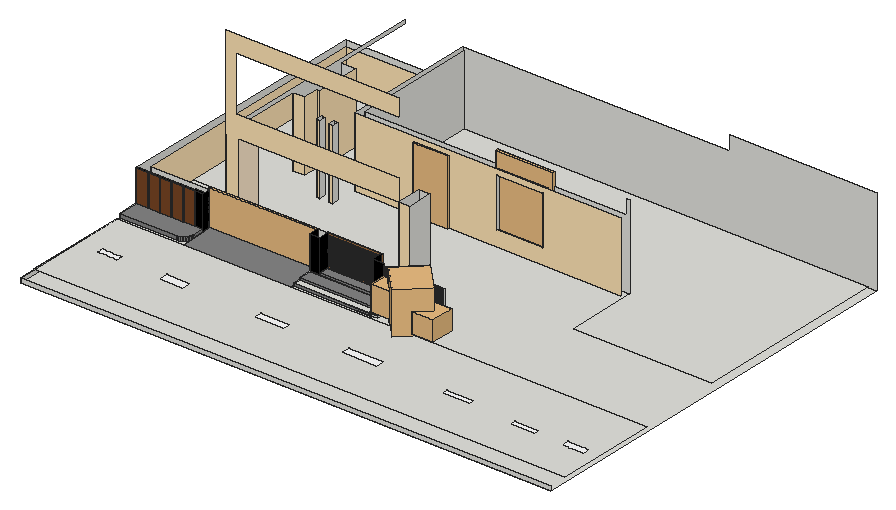
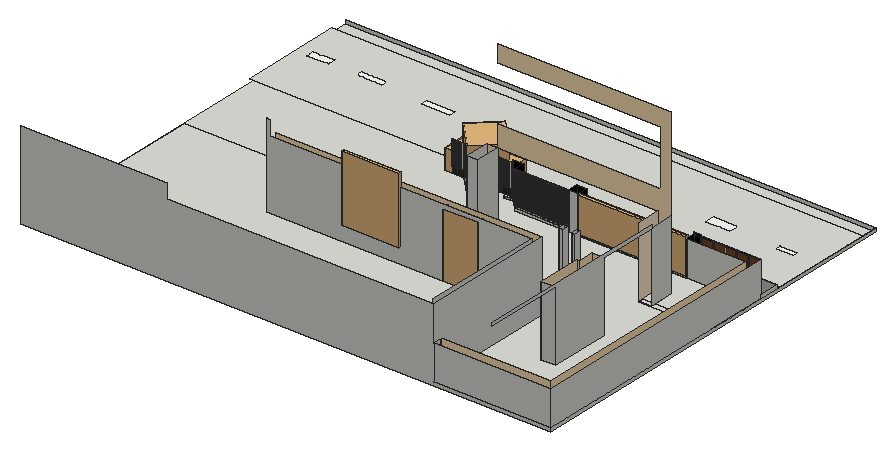
# SketchUp Ruby script. Lengths in inches.
U = 1.inch
M = Sketchup.active_model
def pt(a) = Geom::Point3d.new(a.map { |v| v * U })
def face(e, loops, mat)
  f = e.add_face(loops[0].map { |a| pt(a) })
  loops[1..].each { |l| e.add_face(l.map { |a| pt(a) }).erase! }
  f.material = f.back_material = mat if mat
  f
end
# faces: each face lists its corners as indices into pts; further lists are holes
def faces(e, pts, list, mat = nil) = list.each { |f| face(e, (f[0].is_a?(Array) ? f : [f]).map { |l| l.map { |i| pts[i] } }, mat) }
# xy, xz, yz: faces in a plane at the given z, y or x. An outline is a flat list of corners, or four numbers for a rectangle; further outlines are holes
def ring(l) = l.size == 4 ? [[l[0], l[1]], [l[2], l[1]], [l[2], l[3]], [l[0], l[3]]] : l.each_slice(2).to_a
def flat(e, list, mat, &to3) = list.each { |f| face(e, (f[0].is_a?(Array) ? f : [f]).map { |l| ring(l).map { |u, v| to3.(u, v) } }, mat) }
def xy(e, z, list, mat = nil) = flat(e, list, mat) { |x, y| [x, y, z] }
def xz(e, y, list, mat = nil) = flat(e, list, mat) { |x, z| [x, y, z] }
def yz(e, x, list, mat = nil) = flat(e, list, mat) { |y, z| [x, y, z] }
def lines(e, pts, list) = list.each { |a, b| e.add_line(pt(pts[a]), pt(pts[b])) }
# prism: a flat outline (further loops are holes) pulled along v
def prism(e, loops, v, mat = nil)
  f = face(e, loops, mat); d = Geom::Vector3d.new(v.map { |x| x * U })
  f.pushpull(f.normal.samedirection?(d) ? d.length : -d.length)
end
def box(e, o, s, mat = nil) = prism(e, [[o, [o[0] + s[0], o[1], o[2]], [o[0] + s[0], o[1] + s[1], o[2]], [o[0], o[1] + s[1], o[2]]]], [0, 0, s[2]], mat)
def at(x, y, z, deg = 0) = Geom::Transformation.translation(pt([x, y, z])) * Geom::Transformation.rotation(ORIGIN, Z_AXIS, deg.degrees)
def axes(o, x, y, z) = Geom::Transformation.new([*x, 0, *y, 0, *z, 0, *pt(o).to_a, 1])
def part(name) = M.definitions.add(name)
# library, detail: a bought-in or finely detailed component or shape, given as its bounding box
def library(name, o, s) = part(name).tap { |d| box(d.entities, o, s) }
def detail(e, o, s) = box(e.add_group.entities, o, s)
def put(e, d, t, mat = nil) = e.add_instance(d, t).tap { |i| i.material = mat if mat }
def group(e, t, mat = nil) = e.add_group.tap { |g| g.transformation = t; g.material = mat if mat }.entities
root = M.entities
M.materials.add("Color_000").color = [255, 255, 255]
M.materials.add("Material__1").color = [95, 70, 46]
M.materials.add("Material__2").color = [150, 168, 104]
M.materials.add("[0029_BlanchedAlmond]").color = [255, 235, 205]
M.materials.add("[0032_Moccasin]").color = [255, 228, 181]
M.materials.add("[0136_Charcoal]").color = [35, 35, 35]
M.materials.add("[0137_Black]").color = [0, 0, 0]
M.materials.add("[Tile Grey]").color = [132, 132, 132]
M.materials.add("[Wood Floor Light]").color = [204, 176, 127]
M.materials.add("[Wood Floor]").color = [155, 105, 61]
M.materials.add("[Wood Veneer 01]").color = [120, 70, 37]
M.materials.add("wire_2").color = [244, 244, 244]
M.materials.add("wire_5").color = [232, 232, 232]
c1 = library("Group\#82",[0,0,0],[156.52,4.3,60.67])
c2 = library("door (1)",[38.93,25.48,0],[40,9.94,82.68])
c3 = part("Group\#65")
box(c3.entities,[0,0,0],[1.57,1.97,82.68])
c4 = library("Potted plant on stand",[0,0,0],[37.88,32.09,49.42])
c5 = part("Untitled (5)")
xy(c5.entities,0,[[[158.81,26.5625,306.06,993.3125],[226.57,518.17,239.57,583.92],[225.28,357.51,237.28,411.51],[222.61,182.28,236.36,226.53],[239.71,931.55,251.46,972.3],[233.64,703.93,242.14,755.18],[240.05,835.03,248.8,880.53],[222.04,66.5,231.29,100.5]]])
xy(c5.entities,0,[[222.04,66.5,231.29,100.5],[222.61,182.28,236.36,226.53],[225.28,357.51,237.28,411.51],[226.57,518.17,239.57,583.92],[233.64,703.93,242.14,755.18],
  [240.05,835.03,248.8,880.53],[239.71,931.55,251.46,972.3]],"Color_000")
c6 = library("Cylinder004__30___50_",[-997.48,-49.45,708.79],[29.81,29.81,30.61])
c7 = library("Group\#401",[-996.8,-48.73,736.67],[28.51,28.38,4.73])
c8 = library("Group\#404",[-994.36,-46.95,735.88],[24.38,25.9,6.88])
c9 = library("Group\#388",[-1022.2,-71.69,736.68],[86.94,78.77,45.64])
c10 = library("3 door",[0,0,0],[74.8,3.9375,43.31])
c11 = library("panneau+shadow+blanc+bourdon+naturel",[-47.99,-1.29,1.53],[97.82,5.86,114.18])
c12 = library("Palm",[82.2,-9.29,-2.36],[51.18,55.77,65.42])
c13 = library("Pinch Pot",[-27.95,-27.95,0],[55.9,55.9,47.42])
c14 = library("Group\#386",[-915.9375,-34.5,735.6],[41.04,40.85,6.81])
c15 = library("Group\#403",[-912.1,-32.49,735.82],[33.14,36.63,9.55])
c16 = part("Potted palm")
put(c16.entities,c12,axes([3796.42,-10488.37,43.97],[0,116.51338,0],[-116.51338,0,0],[0,0,116.51338]))
put(c16.entities,c13,axes([1647.67,1801.1875,0],[0,30.58476,0],[-30.58476,0,0],[0,0,45.1095]))
put(c16.entities,c14,axes([32580.48,2279.8125,-23417.78],[34.48768,0,0],[0,34.48768,0],[0,0,34.48768]),"Material__1")
put(c16.entities,c15,axes([32580.48,2279.8125,-23417.78],[34.48768,0,0],[0,34.48768,0],[0,0,34.48768]),"wire_5")
c17 = library("Agrupar\#177",[0,0,0],[36.52,33.08,30.88])
c18 = library("Agrupar\#154",[0,0,0],[41.26,44.6,38.97])
xy(root,0,[[0,84.05,912.4375,784.05]])
xy(root,5.8125,[[0,431.86,124.125,440.22]])
xy(root,6.6875,[[298.71,289.39,114.03,290.125,114.12,311.98,114.13,312.05,114.13,314.23,114.2,333.31,114.27,349.54,298.96,349.54],[298.96,298.09,315.7,332.68],[315.7,298.09,408.98,332.68],[408.98,298.09,430.8,298.09,429.97,299.48,429.25,300.94,428.64,302.43,428.13,303.97,427.73,305.54,427.45,307.14,427.28,308.75,427.22,310.37,427.22,331.81,408.98,331.81],[430.8,298.09,429.97,299.48,429.25,300.94,428.64,302.43,428.13,303.97,427.73,305.54,427.45,307.14,427.28,308.75,427.22,310.37,427.22,331.81,443.3,331.81,443.3,298.09],
  [114.12,311.98,114.13,314.23,114.13,312.05],[298.96,332.68,315.7,349.54],[114.2,333.31,114.27,349.54,114.2,349.54],[114.27,349.54,298.96,349.54,114.27,350.28],[101.6875,397.92,124.125,431.86],
  [101.6875,431.86,124.125,440.22],[666.61,440.22,904.08,440.22,904.08,775.6875,209.98,775.6875,209.98,562.07,666.61,562.07],[101.6875,542.92,121.5,551.1875],[101.6875,551.1875,121.5,569.92]])
xy(root,9.8125,[[298.96,298.09,443.3,298.09,443.3,331.81,430.42,331.81,430.42,310.31,298.96,310.31],[298.96,310.31,315.7,332.68],[315.7,310.31,408.98,332.68],[408.98,310.31,430.42,331.81],[315.7,332.68,408.98,349.54]])
xy(root,12.75,[[0,297.16,98.1875,297.16,100.36,297.31,102.5,297.75,104.55,298.48,106.49,299.49,108.27,300.74,109.87,302.23,111.24,303.93,112.375,305.79,113.25,307.79,113.83,309.89,114.12,311.98,114.13,314.23,114.2,333.31,101.04,333.31,101.04,334.06,100.22,334.06,100.22,333.31,80.99,333.31,80.99,334.06,80.18,334.06,80.18,333.31,60.95,333.31,60.95,334.06,60.13,334.06,60.13,333.31,40.9,333.31,40.9,334.06,40.09,334.06,40.09,333.31,20.86,333.31,20.86,334.06,20.04,334.06,20.04,333.31,0,333.31]],"[Tile Grey]")
xy(root,13.1875,[[315.7,332.68,408.98,349.54]])
xy(root,13.1875,[[298.96,310.31,430.42,310.31,430.42,331.81,408.98,331.81,408.98,332.68,298.96,332.68]],"[Tile Grey]")
xy(root,16.5625,[[315.7,332.68,408.98,349.54]],"[Tile Grey]")
xy(root,32.4,[[446,551.1875,524.68,562.07]])
xz(root,84.05,[[0,0,912.4375,6.6875]])
xz(root,297.16,[[0,6.6875,98.1875,12.75]],"[Tile Grey]")
xz(root,298.09,[[430.8,6.6875,443.3,9.8125]])
xz(root,298.09,[[298.96,6.6875,430.8,9.8125]],"[Tile Grey]")
xz(root,301.86,[[440.93,11.9375,442.89,26],[442.89,11.9375,443.8,26],[443.8,11.9375,445.77,26],[445.77,11.9375,446.68,26],[446.68,11.9375,448.64,26],
  [448.64,11.9375,449.55,26],[449.55,11.9375,451.52,26],[451.52,11.9375,452.37,26],[452.37,11.9375,454.33,26],[454.33,11.9375,455.18,26],
  [455.18,11.9375,457.14,26],[457.14,11.9375,457.99,26],[457.99,11.9375,459.95,26],[459.95,11.9375,460.8,26],[460.8,11.9375,462.77,26],
  [462.77,11.9375,463.62,26],[463.62,11.9375,465.58,26],[465.58,11.9375,466.43,26],[466.43,11.9375,468.39,26],[468.39,11.9375,469.24,26],
  [469.24,11.9375,471.2,26],[471.2,11.9375,472.05,26],[472.05,11.9375,474.02,26],[474.02,11.9375,474.87,26],[474.87,11.9375,476.83,26],
  [476.83,11.9375,477.68,26],[477.68,11.9375,479.64,26],[479.64,11.9375,480.49,26],[480.49,11.9375,482.45,26],[482.45,11.9375,483.3,26],
  [483.3,11.9375,485.27,26],[485.27,11.9375,486.12,26],[486.12,11.9375,488.08,26],[488.08,11.9375,488.93,26],[488.93,11.9375,490.89,26],
  [490.89,11.9375,491.74,26],[491.74,11.9375,493.7,26],[493.7,11.9375,494.55,26],[494.55,11.9375,496.52,26],[496.52,11.9375,497.37,26],
  [497.37,11.9375,499.33,26],[499.33,11.9375,500.18,26],[500.18,11.9375,502.14,26],[502.14,11.9375,502.99,26],[502.99,11.9375,504.95,26],
  [504.95,11.9375,505.8,26],[505.8,11.9375,507.77,26],[507.77,11.9375,508.62,26],[508.62,11.9375,510.58,26],[510.58,11.9375,511.43,26],
  [511.43,11.9375,513.39,26],[513.39,11.9375,514.24,26],[514.24,11.9375,516.2,26],[516.2,11.9375,517.05,26],[517.05,11.9375,519.02,26],
  [519.02,11.9375,520.39,26],[520.39,11.9375,522.35,26],[522.35,11.9375,523.72,26],[523.72,11.9375,525.68,26],[525.68,11.9375,527.06,26],
  [527.06,11.9375,529.02,26],[529.02,11.9375,530.39,26],[530.39,11.9375,532.35,26]],"[Wood Veneer 01]")
xz(root,310.31,[[298.96,9.8125,430.42,13.1875]],"[Tile Grey]")
xz(root,328.88,[[464.85,11.9375,475.34,26]],"[0136_Charcoal]")
xz(root,328.94,[[462.96,11.9375,464.85,26]])
xz(root,328.94,[[452.48,11.9375,462.96,26],[475.34,11.9375,479.46,26]],"[0136_Charcoal]")
xz(root,329,[[430.83,11.9375,434.09,26],[434.09,11.9375,438.21,26],[438.21,11.9375,442.34,26],[442.34,11.9375,446.46,26],[446.46,11.9375,450.59,26],
  [450.59,11.9375,452.48,26],[479.46,11.9375,483.59,26],[483.59,11.9375,487.71,26],[487.71,11.9375,491.84,26],[491.84,11.9375,495.96,26],
  [495.96,11.9375,500.09,26],[500.09,11.9375,504.21,26],[504.21,11.9375,508.34,26],[508.34,11.9375,512.46,26],[512.46,11.9375,516.59,26],
  [516.59,11.9375,520.71,26],[520.71,11.9375,524.84,26],[524.84,11.9375,528.96,26],[528.96,11.9375,533.09,26]],"[0136_Charcoal]")
xz(root,331.81,[[408.98,6.6875,427.22,9.8125],[427.22,6.6875,443.3,9.8125],[408.98,9.8125,427.22,13.1875],[427.22,9.8125,430.42,13.1875]])
xz(root,331.81,[[408.98,13.1875,427.22,70.8125]],"[0137_Black]")
xz(root,332.49,[[468.47,26,471.72,66.6875]],"[Wood Veneer 01]")
xz(root,332.56,[[456.09,26,459.35,66.6875],[464.34,26,467.6,66.6875],[472.59,26,475.85,66.6875]],"[Wood Veneer 01]")
xz(root,332.62,[[427.22,26,430.47,66.6875],[431.34,26,434.6,66.6875],[435.47,26,438.72,66.6875],[439.59,26,442.85,66.6875],[443.72,26,446.97,66.6875],
  [447.84,26,451.1,66.6875],[451.97,26,455.22,66.6875],[460.22,26,463.47,66.6875],[476.72,26,479.97,66.6875],[480.84,26,484.1,66.6875],
  [484.97,26,488.22,66.6875],[489.09,26,492.35,66.6875],[493.22,26,496.47,66.6875],[497.34,26,500.6,66.6875],[501.47,26,504.72,66.6875],
  [505.59,26,508.85,66.6875],[509.72,26,512.97,66.6875],[513.84,26,517.1,66.6875],[517.97,26,521.22,66.6875],[522.09,26,525.35,66.6875],
  [526.22,26,529.47,66.6875]],"[Wood Veneer 01]")
xz(root,332.68,[[298.96,6.6875,315.7,9.8125],[315.7,6.6875,408.98,9.8125],[298.96,9.8125,315.7,13.1875],[315.7,9.8125,408.98,13.1875]])
xz(root,332.68,[[298.96,13.1875,315.7,70.8125]],"[0137_Black]")
xz(root,332.68,[[315.7,13.1875,408.98,16.5625]],"[Tile Grey]")
xz(root,333.31,[[101.04,12.75,114.2,66.6875]],"[0137_Black]")
xz(root,333.31,[[0,12.75,20.04,66.6875],[20.86,12.75,40.09,66.6875],[40.9,12.75,60.13,66.6875],[60.95,12.75,80.18,66.6875],[80.99,12.75,100.22,66.6875],
  [430.47,26,431.34,66.6875],[434.6,26,435.47,66.6875],[438.72,26,439.59,66.6875],[442.85,26,443.72,66.6875],[446.97,26,447.84,66.6875],
  [451.1,26,451.97,66.6875],[455.22,26,456.09,66.6875],[459.35,26,460.22,66.6875],[463.47,26,464.34,66.6875],[467.6,26,468.47,66.6875],
  [471.72,26,472.59,66.6875],[475.85,26,476.72,66.6875],[479.97,26,480.84,66.6875],[484.1,26,484.97,66.6875],[488.22,26,489.09,66.6875],
  [492.35,26,493.22,66.6875],[496.47,26,497.34,66.6875],[500.6,26,501.47,66.6875],[504.72,26,505.59,66.6875],[508.85,26,509.72,66.6875],
  [512.97,26,513.84,66.6875],[517.1,26,517.97,66.6875],[521.22,26,522.09,66.6875],[525.35,26,526.22,66.6875],[529.47,26,530.34,66.6875]],"[Wood Veneer 01]")
xz(root,334.06,[[20.04,12.75,20.86,12.75,20.86,66.6875,40.09,66.6875,40.09,12.75,40.9,12.75,40.9,66.6875,60.13,66.6875,60.13,12.75,60.95,12.75,60.95,66.6875,80.18,66.6875,80.18,12.75,80.99,12.75,80.99,66.6875,100.22,66.6875,100.22,12.75,101.04,12.75,101.04,66.6875,114.2,66.6875,114.2,70.8125,101.1875,70.8125,101.1875,68.25,0,68.25,0,66.6875,20.04,66.6875]],"[0137_Black]")
xz(root,349.54,[[12.79,6.6875,114.2,66.6875],[298.96,6.6875,315.7,70.8125],[315.7,6.6875,408.98,9.8125],[315.7,9.8125,408.98,13.1875],[315.7,13.1875,408.98,16.5625]])
xz(root,397.92,[[101.6875,6.6875,124.125,6.6875,124.125,126.6875,400.76,126.6875,400.76,163.5625,118.89,163.5625,118.89,258.66,400.76,258.66,400.76,287.5625,101.6875,287.5625],[400.76,6.6875,418.84,126.6875]],"[0032_Moccasin]")
xz(root,440.22,[[400.76,6.6875,418.84,126.6875]])
xz(root,506.17,[[171.55,6.6875,177.8,126.6875],[192.11,6.6875,199.48,126.6875]],"[0032_Moccasin]")
xz(root,517.35,[[171.55,6.6875,177.8,126.6875],[192.11,6.6875,199.48,126.6875]])
xz(root,542.92,[[101.6875,6.6875,121.5,126.6875]],"[0032_Moccasin]")
xz(root,551.1875,[[[201.625,6.6875,303.76,6.6875,303.76,118.5,363.88,118.5,363.88,6.6875,660.05,6.6875,660.05,126.6875,201.625,126.6875],[446,32.4,524.68,117.59]]],"[0032_Moccasin]")
xz(root,562.07,[[[209.98,6.6875,209.98,126.6875,660.05,126.6875,660.05,151.4375,666.61,151.4375,666.61,6.6875,363.88,6.6875,363.88,118.5,303.76,118.5,303.76,6.6875],[446,32.4,524.68,117.59]]])
xz(root,569.92,[[121.5,6.6875,126.375,126.6875]],"[0032_Moccasin]")
xz(root,646.79,[[101.6875,6.6875,126.375,126.6875]])
xz(root,768.3,[[12.79,6.6875,201.625,66.6875]],"[0032_Moccasin]")
xz(root,784.05,[[0,0,0,6.6875,201.625,6.6875,201.625,126.6875,660.05,126.6875,660.05,151.4375,912.4375,151.4375,912.4375,0],[0,6.6875,201.625,66.6875]])
yz(root,0,[[84.05,0,84.05,5.8125,440.22,5.8125,440.22,6.6875,784.05,6.6875,784.05,0],[84.05,5.8125,84.05,6.6875,144.1,6.6875,170.97,5.8125],[170.97,5.8125,144.1,6.6875,297.16,6.6875,297.16,12.75,333.31,12.75,333.31,6.6875,431.86,6.6875,431.86,5.8125],[431.86,5.8125,440.22,6.6875],[333.31,6.6875,784.05,66.6875]])
yz(root,12.79,[[349.54,6.6875,768.3,66.6875]],"[0032_Moccasin]")
yz(root,20.04,[[333.31,12.75,334.06,66.6875]])
yz(root,20.86,[[333.31,12.75,334.06,66.6875]])
yz(root,40.09,[[333.31,12.75,334.06,66.6875]])
yz(root,40.9,[[333.31,12.75,334.06,66.6875]])
yz(root,60.13,[[333.31,12.75,334.06,66.6875]])
yz(root,60.95,[[333.31,12.75,334.06,66.6875]])
yz(root,80.18,[[333.31,12.75,334.06,66.6875]])
yz(root,80.99,[[333.31,12.75,334.06,66.6875]])
yz(root,100.22,[[333.31,12.75,334.06,66.6875]])
yz(root,101.04,[[333.31,12.75,334.06,66.6875]])
yz(root,101.6875,[[397.92,6.6875,440.22,126.6875],[542.92,6.6875,542.92,126.6875,440.22,126.6875,440.22,132.6875,784.05,132.6875,784.05,126.6875,646.79,126.6875,646.79,6.6875]])
yz(root,114.2,[[333.31,6.6875,349.54,66.6875]],"[0137_Black]")
yz(root,121.5,[[542.92,6.6875,569.92,126.6875]],"[0032_Moccasin]")
yz(root,124.125,[[431.86,5.8125,440.22,6.6875]])
yz(root,124.125,[[397.92,6.6875,440.22,126.6875]],"[0029_BlanchedAlmond]")
yz(root,126.375,[[569.92,6.6875,646.79,126.6875]],"[0032_Moccasin]")
yz(root,171.55,[[506.17,6.6875,517.35,126.6875]])
yz(root,177.8,[[506.17,6.6875,517.35,126.6875]])
yz(root,192.11,[[506.17,6.6875,517.35,126.6875]])
yz(root,199.48,[[506.17,6.6875,517.35,126.6875]])
yz(root,201.625,[[551.1875,6.6875,551.1875,126.6875,784.05,126.6875,784.05,66.6875,768.3,66.6875,768.3,6.6875]])
yz(root,209.98,[[562.07,6.6875,775.6875,126.6875]])
yz(root,298.96,[[298.09,6.6875,332.68,9.8125],[310.31,9.8125,332.68,13.1875]])
yz(root,298.96,[[332.68,6.6875,349.54,70.8125]],"[0137_Black]")
yz(root,303.76,[[551.1875,6.6875,562.07,118.5]])
yz(root,315.7,[[332.68,6.6875,349.54,9.8125],[332.68,9.8125,349.54,13.1875],[332.68,13.1875,349.54,16.5625]])
yz(root,315.7,[[332.68,16.5625,349.54,70.8125]],"[0137_Black]")
yz(root,363.88,[[551.1875,6.6875,562.07,118.5]])
yz(root,400.76,[[397.92,6.6875,440.22,126.6875]])
yz(root,408.98,[[331.81,6.6875,332.68,9.8125],[331.81,9.8125,332.68,13.1875],[332.68,9.8125,349.54,13.1875],[331.81,13.1875,332.68,17.5625],[332.68,13.1875,349.54,16.5625]])
yz(root,408.98,[[332.68,16.5625,332.68,17.5625,331.81,17.5625,331.81,70.8125,349.54,70.8125,349.54,16.5625]],"[0137_Black]")
yz(root,418.84,[[397.92,6.6875,440.22,126.6875]])
yz(root,427.22,[[310.37,6.6875,331.81,26],[331.81,26,332.62,66.6875]])
yz(root,430.42,[[310.31,9.8125,331.81,13.1875]])
yz(root,430.47,[[332.62,26,333.31,66.6875]])
yz(root,430.83,[[311.3,11.9375,329,26]],"[0136_Charcoal]")
yz(root,431.34,[[332.62,26,333.31,66.6875]])
yz(root,434.6,[[332.62,26,333.31,66.6875]],"[Wood Veneer 01]")
yz(root,435.47,[[332.62,26,333.31,66.6875]])
yz(root,438.72,[[332.62,26,333.31,66.6875]])
yz(root,439.59,[[332.62,26,333.31,66.6875]])
yz(root,442.85,[[332.62,26,333.31,66.6875]])
yz(root,443.3,[[298.09,6.6875,331.81,9.8125]])
yz(root,443.72,[[332.62,26,333.31,66.6875]])
yz(root,446,[[551.1875,32.4,562.07,117.59]])
yz(root,446.97,[[332.62,26,333.31,66.6875]])
yz(root,447.84,[[332.62,26,333.31,66.6875]])
yz(root,451.1,[[332.62,26,333.31,66.6875]])
yz(root,451.97,[[332.62,26,333.31,66.6875]])
yz(root,452.48,[[328.94,11.9375,329,26]])
yz(root,455.22,[[332.62,26,333.31,66.6875]])
yz(root,456.09,[[332.56,26,333.31,66.6875]])
yz(root,459.35,[[332.56,26,333.31,66.6875]])
yz(root,460.22,[[332.62,26,333.31,66.6875]])
yz(root,463.47,[[332.62,26,333.31,66.6875]])
yz(root,464.34,[[332.56,26,333.31,66.6875]])
yz(root,464.85,[[328.88,11.9375,328.94,26]])
yz(root,467.6,[[332.56,26,333.31,66.6875]])
yz(root,468.47,[[332.49,26,333.31,66.6875]])
yz(root,471.72,[[332.49,26,333.31,66.6875]])
yz(root,472.59,[[332.56,26,333.31,66.6875]])
yz(root,475.34,[[328.88,11.9375,328.94,26]])
yz(root,475.85,[[332.56,26,333.31,66.6875]])
yz(root,476.72,[[332.62,26,333.31,66.6875]])
yz(root,479.46,[[328.94,11.9375,329,26]])
yz(root,479.97,[[332.62,26,333.31,66.6875]])
yz(root,480.84,[[332.62,26,333.31,66.6875]])
yz(root,484.1,[[332.62,26,333.31,66.6875]])
yz(root,484.97,[[332.62,26,333.31,66.6875]])
yz(root,488.22,[[332.62,26,333.31,66.6875]])
yz(root,489.09,[[332.62,26,333.31,66.6875]])
yz(root,492.35,[[332.62,26,333.31,66.6875]])
yz(root,493.22,[[332.62,26,333.31,66.6875]])
yz(root,496.47,[[332.62,26,333.31,66.6875]])
yz(root,497.34,[[332.62,26,333.31,66.6875]])
yz(root,500.6,[[332.62,26,333.31,66.6875]])
yz(root,501.47,[[332.62,26,333.31,66.6875]])
yz(root,504.72,[[332.62,26,333.31,66.6875]])
yz(root,505.59,[[332.62,26,333.31,66.6875]])
yz(root,508.85,[[332.62,26,333.31,66.6875]])
yz(root,509.72,[[332.62,26,333.31,66.6875]])
yz(root,512.97,[[332.62,26,333.31,66.6875]])
yz(root,513.84,[[332.62,26,333.31,66.6875]])
yz(root,517.1,[[332.62,26,333.31,66.6875]])
yz(root,517.97,[[332.62,26,333.31,66.6875]])
yz(root,521.22,[[332.62,26,333.31,66.6875]])
yz(root,522.09,[[332.62,26,333.31,66.6875]])
yz(root,524.68,[[551.1875,32.4,562.07,117.59]])
yz(root,525.35,[[332.62,26,333.31,66.6875]])
yz(root,526.22,[[332.62,26,333.31,66.6875]])
yz(root,529.47,[[332.62,26,333.31,66.6875]])
yz(root,530.34,[[332.62,26,333.31,66.6875]])
p = [[298.71,289.39,6.6875],[298.96,349.54,9.6875],[114.27,350.28,9.6875],[114.2,333.31,8.84],[114.13,314.23,7.89],[114.12,311.98,7.78],
  [114.03,290.125,6.6875],[298.96,349.54,6.6875],[114.12,311.98,6.6875],[433.82,294.29,6.6875],[435,293.18,6.6875],[435,293.18,11.9375],
  [433.82,294.29,11.9375],[432.72,295.48,6.6875],[432.72,295.48,11.9375],[431.71,296.75,6.6875],[431.71,296.75,11.9375],[430.8,298.09,6.6875],
  [430.8,298.09,11.9375],[430.8,298.09,9.8125],[98.1875,297.16,6.6875],[100.36,297.31,6.6875],[100.36,297.31,12.75],[98.1875,297.16,12.75],
  [102.5,297.75,6.6875],[102.5,297.75,12.75],[104.55,298.48,6.6875],[104.55,298.48,12.75],[429.97,299.48,6.6875],[429.97,299.48,11.9375],
  [106.49,299.49,6.6875],[106.49,299.49,12.75],[108.27,300.74,6.6875],[108.27,300.74,12.75],[429.25,300.94,6.6875],[429.25,300.94,11.9375],
  [109.87,302.23,6.6875],[109.87,302.23,12.75],[428.64,302.43,6.6875],[428.64,302.43,11.9375],[111.24,303.93,6.6875],[111.24,303.93,12.75],
  [428.13,303.97,6.6875],[428.13,303.97,11.9375],[112.375,305.79,6.6875],[112.375,305.79,12.75],[427.73,305.54,6.6875],[427.73,305.54,11.9375],
  [427.45,307.14,6.6875],[427.45,307.14,11.9375],[113.25,307.79,6.6875],[113.25,307.79,12.75],[427.28,308.75,6.6875],[427.28,308.75,11.9375],
  [113.83,309.89,6.6875],[113.83,309.89,12.75],[427.22,310.37,6.6875],[427.22,310.37,11.9375],[114.12,311.98,12.75],[114.13,314.23,6.6875],
  [114.2,333.31,6.6875],[114.27,349.54,6.6875],[114.27,350.28,6.6875],[114.13,314.23,12.75],[114.2,333.31,12.75],[438.11,302.125,11.9375],
  [439.52,301.93,11.9375],[439.52,301.93,26],[438.11,302.125,26],[440.93,301.86,11.9375],[440.93,301.86,26],[436.74,302.45,11.9375],
  [436.74,302.45,26],[435.39,302.9,11.9375],[435.39,302.9,26],[434.1,303.47,11.9375],[434.1,303.47,26],[432.86,304.16,11.9375],
  [432.86,304.16,26],[431.7,304.96,11.9375],[431.7,304.96,26],[430.61,305.87,11.9375],[430.61,305.87,26],[439.85,305.53,11.9375],
  [438.78,305.68,11.9375],[438.78,305.68,26],[439.85,305.53,26],[441.01,305.48,11.9375],[441.01,305.48,26],[437.73,305.93,11.9375],
  [437.73,305.93,26],[429.61,306.87,11.9375],[429.61,306.87,26],[436.7,306.27,11.9375],[436.7,306.27,26],[435.71,306.71,11.9375],
  [435.71,306.71,26],[434.77,307.24,11.9375],[434.77,307.24,26],[428.7,307.96,11.9375],[428.7,307.96,26],[433.88,307.85,11.9375],
  [433.88,307.85,26],[433.05,308.54,11.9375],[433.05,308.54,26],[427.91,309.13,11.9375],[427.91,309.13,26],[432.28,309.31,11.9375],
  [432.28,309.31,26],[427.22,310.37,26],[431.59,310.14,11.9375],[431.59,310.14,26],[430.98,311.03,11.9375],[430.98,311.03,26],
  [430.83,311.3,11.9375],[430.83,311.3,26],[0,170.97,5.8125],[912.4375,170.97,6.6875]]
faces(root,p,[[0,1,2,3,4,5,6],[20,21,22,23],[21,24,25,22],[24,26,27,25],[26,30,31,27],[30,32,33,31],[32,36,37,33],[36,40,41,37],
  [40,44,45,41],[44,50,51,45],[50,54,55,51],[54,8,5,58,55],[63,4,3,64]],"[Tile Grey]")
faces(root,p,[[0,7,1],[6,5,8],[9,10,11,12],[13,9,12,14],[15,13,14,16],[17,15,16,18,19],[28,17,19,18,29],[34,28,29,35],
  [38,34,35,39],[42,38,39,43],[46,42,43,47],[48,46,47,49],[52,48,49,53],[56,52,53,57],[5,4,59,8],[60,59,4,3],
  [61,60,3,2,62],[1,7,62,2],[58,5,4,63],[83,84,85,86],[87,83,86,88],[84,89,90,85],[89,93,94,90],[93,95,96,94],
  [95,97,98,96],[97,101,102,98],[101,103,104,102],[103,107,108,104],[107,110,111,108],[110,112,113,111],[112,114,115,113]])
faces(root,p,[[65,66,67,68],[66,69,70,67],[71,65,68,72],[73,71,72,74],[75,73,74,76],[77,75,76,78],[79,77,78,80],[81,79,80,82],
  [91,81,82,92],[99,91,92,100],[105,99,100,106],[57,105,106,109]],"[Wood Veneer 01]")
lines(root,p,[[116,117]])
put(root,c1,axes([114.2,347.22,10.14],[1.18039,0,0],[0,1,0],[0,0,1]))
put(root,c2,axes([245.25,512.95,6.6875],[1.50313,0,0],[0,1.36,0],[0,0,1.36]))
g1 = group(root,at(315.7,339.8,16.5625))
g2 = group(g1,at(0,0,0),"[Wood Floor]")
put(g2,c3,axes([34.52,10.4,2.36],[0.78984,0,0],[0,0.67,0],[0,0,0.59911]))
put(g2,c3,axes([54.42,10.4,2.36],[0.78984,0,0],[0,0.67,0],[0,0,0.59911]))
put(g2,c3,axes([86.76,10.4,2.36],[0.78984,0,0],[0,0.67,0],[0,0,0.59911]))
put(g2,c3,axes([81.78,10.4,2.36],[0.78984,0,0],[0,0.67,0],[0,0,0.59911]))
put(g2,c3,axes([44.47,10.4,2.36],[0.78984,0,0],[0,0.67,0],[0,0,0.59911]))
put(g2,c3,axes([61.88,10.4,2.36],[0.78984,0,0],[0,0.67,0],[0,0,0.59911]))
put(g2,c3,axes([56.91,10.4,2.36],[0.78984,0,0],[0,0.67,0],[0,0,0.59911]))
put(g2,c3,axes([24.57,10.4,2.36],[0.78984,0,0],[0,0.67,0],[0,0,0.59911]))
put(g2,c3,axes([69.34,10.4,2.36],[0.78984,0,0],[0,0.67,0],[0,0,0.59911]))
put(g2,c3,axes([37,10.4,2.36],[0.78984,0,0],[0,0.67,0],[0,0,0.59911]))
put(g2,c3,axes([46.96,10.4,2.36],[0.78984,0,0],[0,0.67,0],[0,0,0.59911]))
put(g2,c3,axes([9.64,10.4,2.36],[0.78984,0,0],[0,0.67,0],[0,0,0.59911]))
put(g2,c3,axes([39.49,10.4,2.36],[0.78984,0,0],[0,0.67,0],[0,0,0.59911]))
put(g2,c3,axes([84.27,10.4,2.36],[0.78984,0,0],[0,0.67,0],[0,0,0.59911]))
put(g2,c3,axes([27.05,10.4,2.36],[0.78984,0,0],[0,0.67,0],[0,0,0.59911]))
put(g2,c3,axes([64.37,10.4,2.36],[0.78984,0,0],[0,0.67,0],[0,0,0.59911]))
put(g2,c3,axes([41.98,10.4,2.36],[0.78984,0,0],[0,0.67,0],[0,0,0.59911]))
put(g2,c3,axes([22.08,10.4,2.36],[0.78984,0,0],[0,0.67,0],[0,0,0.59911]))
put(g2,c3,axes([51.93,10.4,2.36],[0.78984,0,0],[0,0.67,0],[0,0,0.59911]))
put(g2,c3,axes([14.62,10.4,2.36],[0.78984,0,0],[0,0.67,0],[0,0,0.59911]))
put(g2,c3,axes([32.03,10.4,2.36],[0.78984,0,0],[0,0.67,0],[0,0,0.59911]))
put(g2,c3,axes([59.39,10.4,2.36],[0.78984,0,0],[0,0.67,0],[0,0,0.59911]))
put(g2,c3,axes([17.1,10.4,2.36],[0.78984,0,0],[0,0.67,0],[0,0,0.59911]))
put(g2,c3,axes([49.44,10.4,2.36],[0.78984,0,0],[0,0.67,0],[0,0,0.59911]))
put(g2,c3,axes([66.86,10.4,2.36],[0.78984,0,0],[0,0.67,0],[0,0,0.59911]))
put(g2,c3,axes([79.3,10.4,2.36],[0.78984,0,0],[0,0.67,0],[0,0,0.59911]))
put(g2,c3,axes([89.25,10.4,2.36],[0.78984,0,0],[0,0.67,0],[0,0,0.59911]))
put(g2,c3,axes([19.59,10.4,2.36],[0.78984,0,0],[0,0.67,0],[0,0,0.59911]))
put(g2,c3,axes([29.54,10.4,2.36],[0.78984,0,0],[0,0.67,0],[0,0,0.59911]))
put(g2,c3,axes([76.81,10.4,2.36],[0.78984,0,0],[0,0.67,0],[0,0,0.59911]))
put(g2,c3,axes([2.18,10.4,2.36],[0.78984,0,0],[0,0.67,0],[0,0,0.59911]))
put(g2,c3,axes([4.66,10.4,2.36],[0.78984,0,0],[0,0.67,0],[0,0,0.59911]))
put(g2,c3,axes([74.32,10.4,2.36],[0.78984,0,0],[0,0.67,0],[0,0,0.59911]))
put(g2,c3,axes([12.13,10.4,2.36],[0.78984,0,0],[0,0.67,0],[0,0,0.59911]))
put(g2,c3,axes([7.15,10.4,2.36],[0.78984,0,0],[0,0.67,0],[0,0,0.59911]))
put(g2,c3,axes([71.83,10.4,2.36],[0.78984,0,0],[0,0.67,0],[0,0,0.59911]))
g3 = group(g1,at(0,9.74,0))
xy(g3,0,[[0,0,93.29,1.98]],"[Wood Floor]")
xy(g3,2.36,[[2.18,0,91.11,1.98]],"[Wood Floor]")
xy(g3,18.28,[[2.18,0,91.11,0.66]],"[Wood Floor]")
xy(g3,18.87,[[2.18,0,91.11,0.66]],"[Wood Floor]")
xy(g3,25.21,[[91.73,1.45,92.35,1.98]],"[Wood Floor]")
xy(g3,25.24,[[0.83,0,1.46,0.53]],"[Wood Floor]")
xy(g3,28.04,[[91.73,1.45,92.35,1.98]],"[Wood Floor]")
xy(g3,28.07,[[0.83,0,1.46,0.53]],"[Wood Floor]")
xy(g3,34.79,[[2.18,0,91.11,0.66]],"[Wood Floor Light]")
xy(g3,35.38,[[2.18,0,91.11,0.66]],"[Wood Floor]")
xy(g3,51.89,[[2.18,0,91.11,1.98]],"[Wood Floor]")
xy(g3,54.25,[[0,0,93.29,1.98]],"[Wood Floor]")
xz(g3,0,[[2.18,18.28,91.11,18.87],[2.18,34.79,91.11,35.38]],"[Wood Floor Light]")
xz(g3,0,[[[0,0,93.29,54.25],[2.18,2.36,91.11,51.89],[0.83,25.24,1.46,28.07]]],"[Wood Floor]")
xz(g3,0.53,[[0.83,25.24,1.46,28.07]],"[Wood Floor]")
xz(g3,0.66,[[2.18,18.28,91.11,18.87],[2.18,34.79,91.11,35.38]],"[Wood Floor]")
xz(g3,1.45,[[91.73,25.21,92.35,28.04]],"[Wood Floor]")
xz(g3,1.98,[[[0,0,93.29,54.25],[2.18,2.36,91.11,51.89],[91.73,25.21,92.35,28.04]]],"[Wood Floor]")
yz(g3,0,[[0,0,1.98,54.25]],"[Wood Floor]")
yz(g3,0.83,[[0,25.24,0.53,28.07]],"[Wood Floor]")
yz(g3,1.46,[[0,25.24,0.53,28.07]],"[Wood Floor]")
yz(g3,2.18,[[0,2.36,1.98,2.36,1.98,51.89,0,51.89,0,35.38,0.66,35.38,0.66,34.79,0,34.79,0,18.87,0.66,18.87,0.66,18.28,0,18.28],[0,18.28,0.66,18.87],[0,34.79,0.66,35.38]],"[Wood Floor]")
yz(g3,91.11,[[0,2.36,0,18.28,0.66,18.28,0.66,18.87,0,18.87,0,34.79,0.66,34.79,0.66,35.38,0,35.38,0,51.89,1.98,51.89,1.98,2.36],[0,18.28,0.66,18.87],[0,34.79,0.66,35.38]],"[Wood Floor]")
yz(g3,91.73,[[1.45,25.21,1.98,28.04]],"[Wood Floor]")
yz(g3,92.35,[[1.45,25.21,1.98,28.04]],"[Wood Floor]")
yz(g3,93.29,[[0,0,1.98,54.25]],"[Wood Floor]")
p = [[4.66,1.98,51.89],[4.66,1.98,2.36]]
lines(g3,p,[[0,1]])
put(root,c4,axes([431.86,298.6,11.9375],[0.87,0,0],[0,0.87,0],[0,0,0.87]))
put(root,c5,axes([-25.07,481.4,7.25],[0,-1.2,0],[0.94382,0,0],[0,0,1]))
put(root,c6,axes([790.8125,325.65,-216.21],[0.3318,0,0],[0,0.3318,0],[0,0,0.3318]),"wire_2")
put(root,c7,axes([790.8125,325.65,-216.21],[0.3318,0,0],[0,0.3318,0],[0,0,0.3318]),"Material__1")
put(root,c8,axes([790.8125,325.65,-216.21],[0.3318,0,0],[0,0.3318,0],[0,0,0.3318]),"wire_5")
put(root,c9,axes([790.8125,325.65,-216.21],[0.3318,0,0],[0,0.3318,0],[0,0,0.3318]),"Material__2")
put(root,c10,axes([443.64,554.9375,28.27],[1.11599,0,0],[0,1,0],[0,0,2.16342]))
put(root,c11,at(485.34,560.375,32.4))
put(root,c16,axes([493.4375,336.59,9.28],[0.0066,-0.00697,0],[-0.00697,-0.0066,0],[0,0,0.0096]),"[Wood Veneer 01]")
put(root,c17,axes([496.84,301.86,18.97],[0.79,0,0],[0,0.79,0],[0,0,0.79]))
put(root,c18,axes([510.08,287.77,10.61],[0.89,0,0],[0,0.89,0],[0,0,0.89]),"[0136_Charcoal]")
